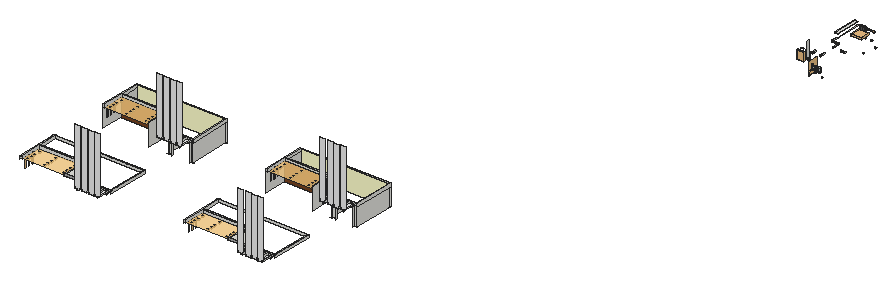
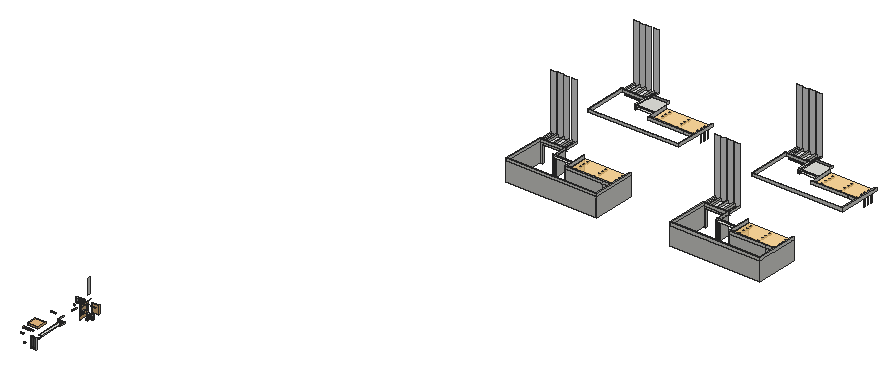
# SketchUp Ruby script. Lengths in inches.
U = 1.inch
M = Sketchup.active_model
def pt(a) = Geom::Point3d.new(a.map { |v| v * U })
def face(e, loops, mat)
  f = e.add_face(loops[0].map { |a| pt(a) })
  loops[1..].each { |l| e.add_face(l.map { |a| pt(a) }).erase! }
  f.material = f.back_material = mat if mat
  f
end
# faces: each face lists its corners as indices into pts; further lists are holes
def faces(e, pts, list, mat = nil) = list.each { |f| face(e, (f[0].is_a?(Array) ? f : [f]).map { |l| l.map { |i| pts[i] } }, mat) }
# xy, xz, yz: faces in a plane at the given z, y or x. An outline is a flat list of corners, or four numbers for a rectangle; further outlines are holes
def ring(l) = l.size == 4 ? [[l[0], l[1]], [l[2], l[1]], [l[2], l[3]], [l[0], l[3]]] : l.each_slice(2).to_a
def flat(e, list, mat, &to3) = list.each { |f| face(e, (f[0].is_a?(Array) ? f : [f]).map { |l| ring(l).map { |u, v| to3.(u, v) } }, mat) }
def xy(e, z, list, mat = nil) = flat(e, list, mat) { |x, y| [x, y, z] }
def xz(e, y, list, mat = nil) = flat(e, list, mat) { |x, z| [x, y, z] }
def yz(e, x, list, mat = nil) = flat(e, list, mat) { |y, z| [x, y, z] }
def lines(e, pts, list) = list.each { |a, b| e.add_line(pt(pts[a]), pt(pts[b])) }
# prism: a flat outline (further loops are holes) pulled along v
def prism(e, loops, v, mat = nil)
  f = face(e, loops, mat); d = Geom::Vector3d.new(v.map { |x| x * U })
  f.pushpull(f.normal.samedirection?(d) ? d.length : -d.length)
end
def box(e, o, s, mat = nil) = prism(e, [[o, [o[0] + s[0], o[1], o[2]], [o[0] + s[0], o[1] + s[1], o[2]], [o[0], o[1] + s[1], o[2]]]], [0, 0, s[2]], mat)
def at(x, y, z, deg = 0) = Geom::Transformation.translation(pt([x, y, z])) * Geom::Transformation.rotation(ORIGIN, Z_AXIS, deg.degrees)
def axes(o, x, y, z) = Geom::Transformation.new([*x, 0, *y, 0, *z, 0, *pt(o).to_a, 1])
def part(name) = M.definitions.add(name)
# library, detail: a bought-in or finely detailed component or shape, given as its bounding box
def library(name, o, s) = part(name).tap { |d| box(d.entities, o, s) }
def detail(e, o, s) = box(e.add_group.entities, o, s)
def put(e, d, t, mat = nil) = e.add_instance(d, t).tap { |i| i.material = mat if mat }
def group(e, t, mat = nil) = e.add_group.tap { |g| g.transformation = t; g.material = mat if mat }.entities
root = M.entities
M.materials.add("6").color = [185, 185, 185]
M.materials.add("WB Frame").color = [245, 245, 245]
M.materials.add("WB Glazing").color = [200, 200, 200]
M.materials["WB Glazing"].alpha = 0.15
M.materials.add("Wood 44").color = [144, 117, 87]
M.materials.add("X22").color = [195, 196, 193]
M.materials.add("[0032_Moccasin]1").color = [255, 228, 181]
M.materials.add("[Carrera Marble]").color = [237, 237, 237]
M.materials.add("[Color E01]").color = [255, 255, 204]
M.materials.add("[Color M03]1").color = [170, 170, 170]
M.materials.add("[Color M08]4").color = [30, 30, 30]
M.materials.add("[Wood Cherry Original]").color = [117, 66, 32]
M.materials.add("[Wood OSB]").color = [255, 207, 129]
M.materials["[Wood OSB]"].alpha = 0.8
M.materials.add("download (88)").color = [169, 176, 150]
c1 = library("Group\#540",[0,0,0],[0.4,67,26])
c2 = part("Window Sliding Main Frame\#3")
prism(c2.entities,[[[35,0,0],[0,0,0],[0,65,0],[35,65,0]],[[1.5,1.5,0],[33.5,1.5,0],[33.5,63.5,0],[1.5,63.5,0]]],[0,0,2.5])
c3 = part("Group428\#1")
xy(c3.entities,0.5,[[3,3,16.75,62]])
c4 = part("Group429\#1")
xy(c4.entities,0.89,[[3,3,16.75,62]])
c5 = part("Window Sliding Casement\#6")
prism(c5.entities,[[[18.25,1.5,0],[1.5,1.5,0],[1.5,63.5,0],[18.25,63.5,0]],[[3,3,0],[16.75,3,0],[16.75,62,0],[3,62,0]]],[0,0,1])
put(c5.entities,c3,at(0,0,0),"WB Glazing")
put(c5.entities,c4,at(0,0,0),"WB Glazing")
c6 = part("Window Sliding Casement\#7")
prism(c6.entities,[[[18.25,1.5,0],[1.5,1.5,0],[1.5,63.5,0],[18.25,63.5,0]],[[3,3,0],[16.75,3,0],[16.75,62,0],[3,62,0]]],[0,0,1])
put(c6.entities,c3,at(0,0,0),"WB Glazing")
put(c6.entities,c4,at(0,0,0),"WB Glazing")
c7 = part("Window Sliding\#3")
put(c7.entities,c2,at(0,0,0),"WB Frame")
put(c7.entities,c5,at(0,0,0),"WB Frame")
put(c7.entities,c6,at(15.25,0,1),"WB Frame")
c8 = library("Group\#467",[0,0,0],[8.82,3.39,0.43])
c9 = library("Group\#465",[0,0,0],[8.82,3.39,0.43])
c10 = library("Group\#488",[0,0,0],[8.82,3.39,0.43])
c11 = library("Group\#466",[0,0,0],[8.82,3.39,0.43])
c12 = library("Group\#541",[0,0,0],[0.4,67,50])
c13 = library("Group\#468",[0,0,0],[8.82,3.39,0.43])
c14 = part("Group\#543")
prism(c14.entities,[[[4.74,0,0],[4.74,0,2.625],[0,0,2.625],[0,0,1.6875],[4.25,0,1.6875],[4.25,0,0]]],[0,1.25,0])
c15 = library("Vase of roses",[-3.61,-2.29,-1.14],[22.21,22.69,31.56])
c16 = part("X1")
xy(c16.entities,0.79,[[292.49,554.16,383.77,683.125],[106.61,647.12,250.85,858.41],[424.25,648.04,568.45,857.91],[293.37,729.03,384.53,857.56]],"X22")
xy(c16.entities,0.79,[[[281.2,542.875,395.06,694.41],[292.49,554.16,383.77,683.125]],[[95.33,635.84,262.14,869.69],[106.61,647.12,250.85,858.41]],[[412.97,636.75,579.74,869.19],[424.25,648.04,568.45,857.91]],[[282.08,717.74,395.82,868.85],[293.37,729.03,384.53,857.56]]],"[Color M08]4")
xz(c16.entities,542.875,[[281.2,-12.48,395.06,0.79]],"X22")
xz(c16.entities,635.84,[[95.33,-12.48,262.14,0.79]],"X22")
xz(c16.entities,636.75,[[412.97,-12.48,579.74,0.79]],"X22")
xz(c16.entities,694.41,[[281.2,-12.48,395.06,0.79]],"X22")
xz(c16.entities,717.74,[[282.08,-12.48,395.82,0.79]],"X22")
xz(c16.entities,868.85,[[282.08,-12.48,395.82,0.79]],"X22")
xz(c16.entities,869.19,[[412.97,-12.48,579.74,0.79]],"X22")
xz(c16.entities,869.69,[[95.33,-12.48,262.14,0.79]],"X22")
yz(c16.entities,95.33,[[635.84,-12.48,869.69,0.79]],"X22")
yz(c16.entities,262.14,[[635.84,-12.48,869.69,0.79]],"[Color M08]4")
yz(c16.entities,281.2,[[542.875,-12.48,694.41,0.79]],"X22")
yz(c16.entities,282.08,[[717.74,-12.48,868.85,0.79]],"X22")
yz(c16.entities,395.06,[[542.875,-12.48,694.41,0.79]],"X22")
yz(c16.entities,395.82,[[717.74,-12.48,868.85,0.79]],"X22")
yz(c16.entities,412.97,[[636.75,-12.48,869.19,0.79]],"X22")
yz(c16.entities,579.74,[[636.75,-12.48,869.19,0.79]],"X22")
c17 = part("Framed Art Print 001")
xy(c17.entities,0,[[-4.59,-0.26,-4.59,0.26,4.59,0.26],[-4.59,-0.26,4.59,0.26,4.59,-0.26]])
xy(c17.entities,12.66,[[-4.59,-0.26,4.59,-0.26,-4.59,0.26],[4.59,-0.26,4.59,0.26,-4.59,0.26]])
xz(c17.entities,-0.26,[[-4.59,0,4.59,0,-4.59,12.66],[4.59,0,4.59,12.66,-4.59,12.66]])
xz(c17.entities,0.26,[[-4.59,0,-4.59,12.66,4.59,12.66],[-4.59,0,4.59,12.66,4.59,0]])
yz(c17.entities,-4.59,[[-0.26,0,-0.26,12.66,0.26,0],[0.26,0,-0.26,12.66,0.26,12.66]])
yz(c17.entities,4.59,[[-0.26,0,0.26,0,-0.26,12.66],[0.26,0,0.26,12.66,-0.26,12.66]])
c18 = library("Group\#528",[0,-11.75,0],[9,47,61.5])
c19 = library("Component\#3",[0,0,0],[1.18,41.92,1.7])
c20 = part("Group\#487")
box(c20.entities,[0,0,0],[4,4,4])
c21 = library("Group\#506",[75.42,83.05,1.23],[65.76,64.05,12.4])
c22 = library("Light+Luminária+Spot+Control",[-53.76,-1.97,-0.51],[47.25,4.73,6.22])
c23 = part("Group\#530")
box(c23.entities,[0,0,0],[0.5,24,0.1])
c24 = library("A$C06767DEF\#1",[-8.3,1.21,0],[7.09,7.09,5.51])
xy(root,115.81,[[647.46,387.84,757.46,394.91],[1695.77,387.84,1805.77,394.91]])
xy(root,120.25,[[647.11,1046.93,757.11,1054],[1695.43,1046.93,1805.43,1054]])
xy(root,126.75,[[208.91,387.84,486.41,528.53],[1257.22,387.84,1534.73,528.53]],"[Wood OSB]")
xy(root,131.1875,[[208.57,1046.93,486.07,1187.62],[1256.88,1046.93,1534.38,1187.62]],"[Wood OSB]")
xy(root,133.625,[[626.68,309.65,641.55,387.84],[657.03,309.65,689.24,387.84],[698.65,309.65,730.86,387.84],[739.28,309.65,761.74,387.84],[1674.99,309.65,1689.86,387.84],
  [1705.34,309.65,1737.55,387.84],[1746.96,309.65,1779.17,387.84],[1787.59,309.65,1810.05,387.84]],"[Carrera Marble]")
xy(root,136.875,[[609.34,309.65,626.68,387.84],[1657.65,309.65,1674.99,387.84]])
xy(root,138,[[500.81,477.09,607.63,494.59],[1549.12,477.09,1655.94,494.59]])
xy(root,138.0625,[[626.34,968.74,641.2,1046.93],[656.68,968.74,688.89,1046.93],[698.31,968.74,730.52,1046.93],[738.93,968.74,761.39,1046.93],[1674.65,968.74,1689.52,1046.93],
  [1705,968.74,1737.2,1046.93],[1746.62,968.74,1778.83,1046.93],[1787.25,968.74,1809.71,1046.93]],"[Carrera Marble]")
xy(root,138.5625,[[609.09,398.1,615.97,448.72],[615.97,398.1,626.68,448.72],[1657.41,398.1,1664.28,448.72],[1664.28,398.1,1674.99,448.72]])
xy(root,139.5,[[761.74,309.65,771.49,387.84],[1810.05,309.65,1819.8,387.84]])
xy(root,141.3125,[[609,968.74,626.34,1046.93],[1657.31,968.74,1674.65,1046.93]])
xy(root,142.4375,[[500.46,1136.18,607.28,1153.68],[1548.77,1136.18,1655.6,1153.68]])
xy(root,143,[[608.75,1057.1875,615.625,1107.8125],[615.625,1057.1875,626.34,1107.8125],[1657.0625,1057.1875,1663.9375,1107.8125],[1663.9375,1057.1875,1674.65,1107.8125]])
xy(root,143.9375,[[761.39,968.74,771.14,1046.93],[1809.71,968.74,1819.45,1046.93]])
xy(root,144.3125,[[497.6,365.47,497.6,387.84,499.53,387.84,499.53,477.09,609.09,477.09,609.09,365.47],[609.09,365.47,626.68,387.84],[1545.92,365.47,1545.92,387.84,1547.84,387.84,1547.84,477.09,1657.41,477.09,1657.41,365.47],[1657.41,365.47,1674.99,387.84],[609.09,387.84,626.68,387.84,626.68,394.91,616.45,394.91,616.45,477.09,609.09,477.09],
  [1657.41,387.84,1674.99,387.84,1674.99,394.91,1664.77,394.91,1664.77,477.09,1657.41,477.09],[616.45,394.91,626.68,477.09],[1664.77,394.91,1674.99,477.09],[607.63,477.09,616.45,494.59],[1655.94,477.09,1664.77,494.59]])
xz(root,309.65,[[626.68,133.625,641.55,133.625,641.55,502.82,609.34,502.82,609.34,136.875,626.68,136.875],[657.03,133.625,689.24,502.82],[698.65,133.625,730.86,502.82],[739.28,133.625,761.74,133.625,761.74,139.5,771.49,139.5,771.49,502.82,739.28,502.82],[1674.99,133.625,1689.86,133.625,1689.86,502.82,1657.65,502.82,1657.65,136.875,1674.99,136.875],
  [1705.34,133.625,1737.55,502.82],[1746.96,133.625,1779.17,502.82],[1787.59,133.625,1810.05,133.625,1810.05,139.5,1819.8,139.5,1819.8,502.82,1787.59,502.82]],"[Carrera Marble]")
xz(root,365.47,[[609.09,144.3125,626.68,144.9375],[1657.41,144.3125,1674.99,144.9375]])
xz(root,365.47,[[497.6,144.3125,609.09,157.5],[1545.92,144.3125,1657.41,157.5]],"[Color M03]1")
xz(root,387.84,[[626.68,133.625,641.55,144.3125],[657.03,133.625,689.24,144.3125],[698.65,133.625,730.86,144.3125],[739.28,133.625,761.74,133.625,761.74,139.5,771.49,139.5,771.49,144.3125,739.28,144.3125],[1674.99,133.625,1689.86,144.3125],
  [1705.34,133.625,1737.55,144.3125],[1746.96,133.625,1779.17,144.3125],[1787.59,133.625,1810.05,133.625,1810.05,139.5,1819.8,139.5,1819.8,144.3125,1787.59,144.3125],[609.34,136.875,626.68,144.3125],[1657.65,136.875,1674.99,144.3125],
  [609.09,144.3125,609.34,144.9375],[609.34,144.3125,626.68,144.9375],[626.68,144.3125,641.55,144.9375],[641.55,144.3125,657.03,144.9375],[689.24,144.3125,698.65,144.9375],
  [730.86,144.3125,739.28,144.9375],[771.49,144.3125,782.78,144.9375],[1657.41,144.3125,1657.65,144.9375],[1657.65,144.3125,1674.99,144.9375],[1674.99,144.3125,1689.86,144.9375],
  [1689.86,144.3125,1705.34,144.9375],[1737.55,144.3125,1746.96,144.9375],[1779.17,144.3125,1787.59,144.9375],[1819.8,144.3125,1831.09,144.9375]])
xz(root,394.91,[[493.2,126.75,497.6,144.3125],[616.45,126.75,775.16,144.3125],[1541.52,126.75,1545.92,144.3125],[1664.77,126.75,1823.47,144.3125]])
xz(root,477.09,[[499.53,126.75,500.81,144.3125],[607.63,126.75,609.09,144.3125],[609.09,126.75,626.68,144.3125],[1547.84,126.75,1549.12,144.3125],[1655.94,126.75,1657.41,144.3125],
  [1657.41,126.75,1674.99,144.3125],[500.81,138,607.63,144.3125],[1549.12,138,1655.94,144.3125]])
xz(root,494.59,[[499.53,126.75,500.81,144.3125],[607.63,126.75,616.45,144.3125],[1547.84,126.75,1549.12,144.3125],[1655.94,126.75,1664.77,144.3125]])
xz(root,528.53,[[208.91,126.75,493.2,144.3125],[1257.22,126.75,1541.52,144.3125]])
xz(root,538.16,[[208.91,126.75,262.79,144.3125],[262.79,126.75,499.53,144.3125],[1257.22,126.75,1311.1,144.3125],[1311.1,126.75,1547.84,144.3125]])
xz(root,659.09,[[200.03,126.75,782.78,144.3125],[1248.34,126.75,1831.09,144.3125],[200.03,144.3125,782.78,144.9375],[1248.34,144.3125,1831.09,144.9375]])
xz(root,968.74,[[626.34,138.0625,641.2,138.0625,641.2,507.25,609,507.25,609,141.3125,626.34,141.3125],[656.68,138.0625,688.89,507.25],[698.31,138.0625,730.52,507.25],[738.93,138.0625,761.39,138.0625,761.39,143.9375,771.14,143.9375,771.14,507.25,738.93,507.25],[1674.65,138.0625,1689.52,138.0625,1689.52,507.25,1657.31,507.25,1657.31,141.3125,1674.65,141.3125],
  [1705,138.0625,1737.2,507.25],[1746.62,138.0625,1778.83,507.25],[1787.25,138.0625,1809.71,138.0625,1809.71,143.9375,1819.45,143.9375,1819.45,507.25,1787.25,507.25]],"[Carrera Marble]")
xz(root,1046.93,[[626.34,138.0625,641.2,148.75],[656.68,138.0625,688.89,148.75],[698.31,138.0625,730.52,148.75],[738.93,138.0625,761.39,138.0625,761.39,143.9375,771.14,143.9375,771.14,148.75,738.93,148.75],[1674.65,138.0625,1689.52,148.75],
  [1705,138.0625,1737.2,148.75],[1746.62,138.0625,1778.83,148.75],[1787.25,138.0625,1809.71,138.0625,1809.71,143.9375,1819.45,143.9375,1819.45,148.75,1787.25,148.75],[609,141.3125,626.34,148.75],[1657.31,141.3125,1674.65,148.75]])
xz(root,1054,[[616.11,11.1875,616.11,131.1875,774.8125,131.1875,774.8125,11.1875,757.11,11.1875,757.11,120.25,647.11,120.25,647.11,11.1875],[1664.42,11.1875,1664.42,131.1875,1823.125,131.1875,1823.125,11.1875,1805.43,11.1875,1805.43,120.25,1695.43,120.25,1695.43,11.1875],[492.86,131.1875,497.26,148.75],[616.11,131.1875,774.8125,148.75],[1541.17,131.1875,1545.57,148.75],
  [1664.42,131.1875,1823.125,148.75]])
xz(root,1136.18,[[499.1875,11.1875,500.46,131.1875],[607.28,11.1875,608.75,131.1875],[608.75,11.1875,626.34,131.1875],[1547.5,11.1875,1548.77,131.1875],[1655.6,11.1875,1657.0625,131.1875],
  [1657.0625,11.1875,1674.65,131.1875],[499.1875,131.1875,500.46,148.75],[607.28,131.1875,608.75,148.75],[608.75,131.1875,626.34,148.75],[1547.5,131.1875,1548.77,148.75],
  [1655.6,131.1875,1657.0625,148.75],[1657.0625,131.1875,1674.65,148.75],[500.46,142.4375,607.28,148.75],[1548.77,142.4375,1655.6,148.75]])
xz(root,1153.68,[[499.1875,11.1875,500.46,131.1875],[607.28,11.1875,616.11,131.1875],[1547.5,11.1875,1548.77,131.1875],[1655.6,11.1875,1664.42,131.1875],[499.1875,131.1875,500.46,148.75],
  [607.28,131.1875,616.11,148.75],[1547.5,131.1875,1548.77,148.75],[1655.6,131.1875,1664.42,148.75]])
xz(root,1187.62,[[486.07,11.1875,492.86,131.1875],[1534.38,11.1875,1541.17,131.1875],[208.57,131.1875,492.86,148.75],[1256.88,131.1875,1541.17,148.75]])
xz(root,1187.62,[[208.57,11.1875,486.07,131.1875],[1256.88,11.1875,1534.38,131.1875]],"[Wood Cherry Original]")
xz(root,1197.25,[[208.57,11.1875,262.44,131.1875],[262.44,11.1875,499.1875,131.1875],[1256.88,11.1875,1310.75,131.1875],[1310.75,11.1875,1547.5,131.1875],[208.57,131.1875,262.44,148.75],
  [262.44,131.1875,499.1875,148.75],[1256.88,131.1875,1310.75,148.75],[1310.75,131.1875,1547.5,148.75]])
xz(root,1311.11,[[208.57,11.1875,774.8125,148.75],[1256.88,11.1875,1823.125,148.75]],"[Color E01]")
xz(root,1318.18,[[199.6875,11.1875,782.4375,131.1875],[1248,11.1875,1830.75,131.1875],[199.6875,131.1875,782.4375,148.75],[1248,131.1875,1830.75,148.75]])
yz(root,199.6875,[[1046.93,11.1875,1318.18,131.1875],[1046.93,131.1875,1318.18,148.75]])
yz(root,200.03,[[387.84,126.75,659.09,144.3125],[387.84,144.3125,659.09,144.9375]])
yz(root,208.57,[[1197.25,11.1875,1311.11,131.1875],[1054,131.1875,1187.62,148.75],[1197.25,131.1875,1311.11,148.75]])
yz(root,208.91,[[394.91,126.75,528.53,144.3125],[538.16,126.75,652.02,144.3125]])
yz(root,492.86,[[1054,131.1875,1187.62,148.75]])
yz(root,493.2,[[394.91,126.75,528.53,144.3125]])
yz(root,497.6,[[365.47,144.3125,387.84,157.5]])
yz(root,499.1875,[[1046.93,11.1875,1136.18,148.75],[1153.68,11.1875,1197.25,148.75]])
yz(root,500.46,[[1136.18,11.1875,1153.68,142.4375],[1136.18,142.4375,1153.68,148.75]])
yz(root,500.81,[[477.09,138,494.59,144.3125]])
yz(root,607.28,[[1136.18,142.4375,1153.68,148.75]])
yz(root,607.63,[[477.09,138,494.59,144.3125]])
yz(root,609,[[968.74,141.3125,1046.93,149.375]])
yz(root,609.09,[[365.47,144.3125,387.84,144.9375],[387.84,144.3125,389.4,144.9375]])
yz(root,609.34,[[309.65,136.875,387.84,144.9375]])
yz(root,616.11,[[1054,11.1875,1153.68,131.1875],[1054,131.1875,1153.68,148.75]])
yz(root,616.45,[[394.91,126.75,494.59,144.3125]])
yz(root,626.34,[[968.74,138.0625,1000.12,141.3125],[1000.12,138.0625,1046.93,141.3125],[1046.93,138.0625,1048.49,141.3125],[1000.12,141.3125,1046.93,141.3125,1046.93,148.75,1024.56,148.75,1024.56,149.375,1000.12,149.375],[1046.93,141.3125,1048.49,148.75]])
yz(root,626.68,[[309.65,133.625,341.03,136.875],[341.03,133.625,387.84,136.875],[387.84,133.625,389.4,136.875],[341.03,136.875,387.84,136.875,387.84,144.3125,365.47,144.3125,365.47,144.9375,341.03,144.9375],[387.84,136.875,389.4,144.3125],
  [365.47,144.3125,387.84,144.9375],[387.84,144.3125,389.4,144.9375]])
yz(root,641.2,[[968.74,138.0625,1046.93,149.375]])
yz(root,641.55,[[309.65,133.625,387.84,144.9375]])
yz(root,647.11,[[1046.93,11.1875,1054,120.25]])
yz(root,656.68,[[968.74,138.0625,1046.93,149.375]])
yz(root,657.03,[[309.65,133.625,387.84,144.9375]])
yz(root,688.89,[[968.74,138.0625,1046.93,149.375]])
yz(root,689.24,[[309.65,133.625,387.84,144.9375]])
yz(root,698.31,[[968.74,138.0625,1046.93,149.375]])
yz(root,698.65,[[309.65,133.625,387.84,144.9375]])
yz(root,730.52,[[968.74,138.0625,1046.93,149.375]])
yz(root,730.86,[[309.65,133.625,387.84,144.9375]])
yz(root,738.93,[[968.74,138.0625,1046.93,149.375]])
yz(root,739.28,[[309.65,133.625,387.84,144.9375]])
yz(root,757.11,[[1046.93,11.1875,1054,120.25]])
yz(root,761.39,[[968.74,138.0625,1046.93,143.9375]])
yz(root,761.74,[[309.65,133.625,387.84,139.5]])
yz(root,771.14,[[968.74,143.9375,1046.93,149.375]])
yz(root,771.49,[[309.65,139.5,387.84,144.9375]])
yz(root,774.8125,[[1054,11.1875,1311.11,131.1875],[1054,131.1875,1311.11,148.75]])
yz(root,775.16,[[394.91,126.75,652.02,144.3125]])
yz(root,782.4375,[[1046.93,131.1875,1318.18,148.75]])
yz(root,782.78,[[387.84,126.75,659.09,144.3125],[387.84,144.3125,659.09,144.9375]])
yz(root,1248,[[1046.93,11.1875,1318.18,131.1875],[1046.93,131.1875,1318.18,148.75]])
yz(root,1248.34,[[387.84,126.75,659.09,144.3125],[387.84,144.3125,659.09,144.9375]])
yz(root,1256.88,[[1197.25,11.1875,1311.11,131.1875],[1054,131.1875,1187.62,148.75],[1197.25,131.1875,1311.11,148.75]])
yz(root,1257.22,[[394.91,126.75,528.53,144.3125],[538.16,126.75,652.02,144.3125]])
yz(root,1541.17,[[1054,131.1875,1187.62,148.75]])
yz(root,1541.52,[[394.91,126.75,528.53,144.3125]])
yz(root,1545.92,[[365.47,144.3125,387.84,157.5]])
yz(root,1547.5,[[1046.93,11.1875,1136.18,148.75],[1153.68,11.1875,1197.25,148.75]])
yz(root,1548.77,[[1136.18,11.1875,1153.68,142.4375],[1136.18,142.4375,1153.68,148.75]])
yz(root,1549.12,[[477.09,138,494.59,144.3125]])
yz(root,1655.6,[[1136.18,142.4375,1153.68,148.75]])
yz(root,1655.94,[[477.09,138,494.59,144.3125]])
yz(root,1657.31,[[968.74,141.3125,1046.93,149.375]])
yz(root,1657.41,[[365.47,144.3125,387.84,144.9375],[387.84,144.3125,389.4,144.9375]])
yz(root,1657.65,[[309.65,136.875,387.84,144.9375]])
yz(root,1664.42,[[1054,11.1875,1153.68,131.1875],[1054,131.1875,1153.68,148.75]])
yz(root,1664.77,[[394.91,126.75,494.59,144.3125]])
yz(root,1674.65,[[968.74,138.0625,1000.12,141.3125],[1000.12,138.0625,1046.93,141.3125],[1046.93,138.0625,1048.49,141.3125],[1000.12,141.3125,1046.93,141.3125,1046.93,148.75,1024.56,148.75,1024.56,149.375,1000.12,149.375],[1046.93,141.3125,1048.49,148.75]])
yz(root,1674.99,[[309.65,133.625,341.03,136.875],[341.03,133.625,387.84,136.875],[387.84,133.625,389.4,136.875],[341.03,136.875,387.84,136.875,387.84,144.3125,365.47,144.3125,365.47,144.9375,341.03,144.9375],[387.84,136.875,389.4,144.3125],
  [365.47,144.3125,387.84,144.9375],[387.84,144.3125,389.4,144.9375]])
yz(root,1689.52,[[968.74,138.0625,1046.93,149.375]])
yz(root,1689.86,[[309.65,133.625,387.84,144.9375]])
yz(root,1695.43,[[1046.93,11.1875,1054,120.25]])
yz(root,1705,[[968.74,138.0625,1046.93,149.375]])
yz(root,1705.34,[[309.65,133.625,387.84,144.9375]])
yz(root,1737.2,[[968.74,138.0625,1046.93,149.375]])
yz(root,1737.55,[[309.65,133.625,387.84,144.9375]])
yz(root,1746.62,[[968.74,138.0625,1046.93,149.375]])
yz(root,1746.96,[[309.65,133.625,387.84,144.9375]])
yz(root,1778.83,[[968.74,138.0625,1046.93,149.375]])
yz(root,1779.17,[[309.65,133.625,387.84,144.9375]])
yz(root,1787.25,[[968.74,138.0625,1046.93,149.375]])
yz(root,1787.59,[[309.65,133.625,387.84,144.9375]])
yz(root,1805.43,[[1046.93,11.1875,1054,120.25]])
yz(root,1809.71,[[968.74,138.0625,1046.93,143.9375]])
yz(root,1810.05,[[309.65,133.625,387.84,139.5]])
yz(root,1819.45,[[968.74,143.9375,1046.93,149.375]])
yz(root,1819.8,[[309.65,139.5,387.84,144.9375]])
yz(root,1823.125,[[1054,11.1875,1311.11,131.1875],[1054,131.1875,1311.11,148.75]])
yz(root,1823.47,[[394.91,126.75,652.02,144.3125]])
yz(root,1830.75,[[1046.93,131.1875,1318.18,148.75]])
yz(root,1831.09,[[387.84,126.75,659.09,144.3125],[387.84,144.3125,659.09,144.9375]])
p = [[609.09,387.84,126.75],[626.68,387.84,126.75],[208.91,394.91,144.3125],[208.91,387.84,144.3125],[493.2,394.91,126.75],[493.2,387.84,126.75],
  [497.6,394.91,144.3125],[497.6,387.84,144.3125],[1257.22,394.91,144.3125],[1257.22,387.84,144.3125],[1657.41,387.84,126.75],[1674.99,387.84,126.75],
  [1541.52,394.91,126.75],[1541.52,387.84,126.75],[1545.92,394.91,144.3125],[1545.92,387.84,144.3125],[782.4375,1054,11.1875],[774.8125,1054,11.1875],
  [262.44,1197.25,11.1875],[262.44,1187.62,11.1875],[782.4375,1311.11,11.1875],[774.8125,1311.11,11.1875],[782.4375,1318.18,11.1875],[608.75,1046.93,11.1875],
  [626.34,1046.93,11.1875],[608.75,1046.93,131.1875],[626.34,1046.93,131.1875],[492.86,1054,131.1875],[492.86,1046.93,131.1875],[1830.75,1054,11.1875],
  [1823.125,1054,11.1875],[1310.75,1197.25,11.1875],[1310.75,1187.62,11.1875],[1830.75,1311.11,11.1875],[1830.75,1318.18,11.1875],[1657.0625,1046.93,11.1875],
  [1674.65,1046.93,11.1875],[1823.125,1311.11,11.1875],[1657.0625,1046.93,131.1875],[1674.65,1046.93,131.1875],[1541.17,1054,131.1875],[1541.17,1046.93,131.1875]]
lines(root,p,[[0,1],[2,3],[4,5],[6,7],[8,9],[10,11],[12,13],[14,15],[16,17],[18,19],[20,21],[20,22],
  [23,24],[25,26],[27,28],[29,30],[31,32],[33,34],[35,36],[33,37],[38,39],[40,41]])
put(root,c1,at(2620.7,3681.75,8))
put(root,c1,axes([2620.76,3685.75,12],[0.85,0,0],[0,0.8806,0],[0,0,0.69231]))
put(root,c7,axes([2622.1,4135.25,22],[-1,0,0],[0,0,1],[0,1,0]))
put(root,c8,axes([2709.35,4002.67,26.4],[1,0,0],[0,0,1],[0,1,0]),"Wood 44")
put(root,c9,axes([2662.49,4128.75,27.19],[1,0,0],[0,0,1],[0,-1,0]),"Wood 44")
put(root,c10,axes([2564.28,3755.94,30],[1,0,0],[0,0,1],[0,-1,0]))
put(root,c11,axes([2708.28,3675.94,30],[1,0,0],[0,0,1],[0,-1,0]),"Wood 44")
put(root,c12,at(2620.7,3681.75,35))
put(root,c13,axes([2731.52,4069.75,35.14],[1,0,0],[0,0,1],[0,1,0]),"Wood 44")
put(root,c8,axes([2732.92,4070.75,35.72],[1,0,0],[0,0,1],[0,1,0]),"Wood 44")
put(root,c14,at(2616.36,3725.98,36.31))
put(root,c14,at(2616.36,3703.1,36.31))
put(root,c15,axes([2613.87,3711.5,38.51],[0.3886,0,0],[0,0.3886,0],[0,0,0.3886]))
g1 = group(root,at(2615.1,3700.75,38.17))
prism(g1,[[[5.95,29,0],[5.95,0,0],[1.7,0,0],[1.48,0.02,0],[1.26,0.07,0],[1.05,0.15,0],[0.85,0.27,0],[0.67,0.41,0],[0.5,0.59,0],[0.35,0.78,0],[0.23,1,0],[0.13,1.23,0],[0.06,1.48,0],[0.01,1.74,0],[0,2,0],[0,27,0],[0.01,27.26,0],[0.06,27.52,0],[0.13,27.77,0],[0.23,28,0],[0.35,28.22,0],[0.5,28.41,0],[0.67,28.59,0],[0.85,28.73,0],[1.05,28.85,0],[1.26,28.93,0],[1.48,28.98,0],[1.7,29,0]]],[0,0,0.52])
g2 = group(root,at(2620.6,3688.75,41.7))
yz(g2,0,[[0.5,0.5,52.5,35.5]],"WB Glazing")
g3 = group(g2,at(0,0,0))
xy(g3,0,[[0,0,0.5,53]],"6")
xy(g3,0.5,[[0,0.5,0.25,52.5]],"6")
xy(g3,35.5,[[0,0.5,0.25,52.5]],"6")
xy(g3,36,[[0,0,0.5,53]],"6")
xz(g3,0,[[0,0,0.5,36]],"6")
xz(g3,0.5,[[0,0.5,0.25,35.5]],"6")
xz(g3,52.5,[[0,0.5,0.25,35.5]],"6")
xz(g3,53,[[0,0,0.5,36]],"6")
yz(g3,0,[[[0,0,53,36],[0.5,0.5,52.5,35.5]]],"6")
yz(g3,0.5,[[0,0,53,36]],"6")
g4 = group(g2,at(0.25,0.5,0.5),"WB Glazing")
yz(g4,0,[[0,0,52,35]],"download (88)")
put(root,c16,axes([2631.17,3676.52,-21.4],[0.12,0,0],[0,0,0.12],[0,-0.018,0]))
put(root,c17,axes([2558.54,3755.55,45.375],[2.19,0,0],[0,0.7884,0],[0,0,2.19]))
put(root,c17,axes([2533.67,3755.55,45.375],[2.19,0,0],[0,0.7884,0],[0,0,2.19]))
put(root,c18,axes([2534.41,3716.78,108.92],[0,-1.33292,0],[1,0,0],[0,0,-0.782]))
put(root,c19,axes([208.91,414.82,130.83],[0,-1,0],[0,0,-1.54],[1,0,0]))
put(root,c19,axes([208.91,442.82,130.83],[0,-1,0],[0,0,-1.54],[1,0,0]))
put(root,c19,axes([208.91,472.57,130.83],[0,-1,0],[0,0,-1.54],[1,0,0]))
put(root,c19,axes([1257.22,414.82,130.83],[0,-1,0],[0,0,-1.54],[1,0,0]))
put(root,c19,axes([1257.22,442.82,130.83],[0,-1,0],[0,0,-1.54],[1,0,0]))
put(root,c19,axes([1257.22,472.57,130.83],[0,-1,0],[0,0,-1.54],[1,0,0]))
put(root,c19,axes([208.57,1073.91,135.27],[0,-1,0],[0,0,-1.54],[1,0,0]))
put(root,c19,axes([208.57,1101.91,135.27],[0,-1,0],[0,0,-1.54],[1,0,0]))
put(root,c19,axes([208.57,1131.66,135.27],[0,-1,0],[0,0,-1.54],[1,0,0]))
put(root,c19,axes([1256.88,1073.91,135.27],[0,-1,0],[0,0,-1.54],[1,0,0]))
put(root,c19,axes([1256.88,1101.91,135.27],[0,-1,0],[0,0,-1.54],[1,0,0]))
put(root,c19,axes([1256.88,1131.66,135.27],[0,-1,0],[0,0,-1.54],[1,0,0]))
put(root,c9,axes([2672.34,4131.75,79.41],[1,0,0],[0,0,1],[0,-1,0]),"Wood 44")
put(root,c20,axes([2581.1,3918.75,83],[9.25,0,0],[0,1.5,0],[0,0,1]))
put(root,c20,axes([2674.06,3868.75,83],[6.76,0,0],[0,1.5,0],[0,0,1]))
put(root,c20,axes([2621.1,3765.75,83],[1.5,0,0],[0,9,0],[0,0,1]))
put(root,c20,axes([2621.1,3874.75,83],[1.25,0,0],[0,9.25,0],[0,0,1]))
put(root,c20,axes([2573.1,3764.75,83],[1.5,0,0],[0,7,0],[0,0,1]))
put(root,c20,axes([2573.1,3928.75,83],[1.5,0,0],[0,7,0],[0,0,1]))
g5 = group(root,at(2578.1,3967.75,84.2))
box(g5,[0,0,0],[0.75,161,1.1])
put(root,c21,at(2555.1,3924.75,94),"Wood 44")
put(root,c22,at(2700.23,4106.59,98.1875))
g6 = group(root,at(2555.1,3967.75,0))
g7 = group(g6,at(0.125,0,104.0625))
xy(g7,0,[[0,0,23.625,161]])
xy(g7,3.9375,[[0,0,23.625,161]])
xz(g7,0,[[0,0,23.625,3.9375]])
xz(g7,161,[[0,0,23.625,3.9375]])
yz(g7,0,[[0,0,161,3.9375]])
yz(g7,23.625,[[0,0,161,3.9375]],"Wood 44")
put(root,c23,axes([2598.6,3686.75,109.9],[1,0,0],[0,2.375,0],[0,0,1]),"[0032_Moccasin]1")
put(root,c23,axes([2523.1,3737.78,109.9],[0,-1,0],[3.66667,0,0],[0,0,1]),"[0032_Moccasin]1")
g8 = group(root,at(2624.1,3657.75,120.91))
yz(g8,0,[[0,0,18,92.85]])
put(root,c24,at(235.46,497.86,121.24))
put(root,c24,at(235.46,461.74,121.24))
put(root,c24,at(235.46,435.43,121.24))
put(root,c24,at(235.46,407.55,121.24))
put(root,c24,at(342.15,407.55,121.24))
put(root,c24,at(342.15,497.86,121.24))
put(root,c24,at(342.15,435.43,121.24))
put(root,c24,at(342.15,461.74,121.24))
put(root,c24,at(462.77,407.55,121.24))
put(root,c24,at(462.77,497.86,121.24))
put(root,c24,at(462.77,435.43,121.24))
put(root,c24,at(462.77,461.74,121.24))
put(root,c24,at(1390.46,407.55,121.24))
put(root,c24,at(1283.77,407.55,121.24))
put(root,c24,at(1283.77,497.86,121.24))
put(root,c24,at(1283.77,435.43,121.24))
put(root,c24,at(1390.46,497.86,121.24))
put(root,c24,at(1390.46,435.43,121.24))
put(root,c24,at(1390.46,461.74,121.24))
put(root,c24,at(1283.77,461.74,121.24))
put(root,c24,at(1511.09,461.74,121.24))
put(root,c24,at(1511.09,435.43,121.24))
put(root,c24,at(1511.09,407.55,121.24))
put(root,c24,at(1511.09,497.86,121.24))
put(root,c24,at(341.8,1066.64,125.68))
put(root,c24,at(235.12,1066.64,125.68))
put(root,c24,at(235.12,1156.95,125.68))
put(root,c24,at(235.12,1094.52,125.68))
put(root,c24,at(341.8,1156.95,125.68))
put(root,c24,at(341.8,1094.52,125.68))
put(root,c24,at(341.8,1120.83,125.68))
put(root,c24,at(235.12,1120.83,125.68))
put(root,c24,at(462.43,1120.83,125.68))
put(root,c24,at(462.43,1094.52,125.68))
put(root,c24,at(462.43,1066.64,125.68))
put(root,c24,at(462.43,1156.95,125.68))
put(root,c24,at(1510.74,1094.52,125.68))
put(root,c24,at(1510.74,1156.95,125.68))
put(root,c24,at(1510.74,1066.64,125.68))
put(root,c24,at(1283.43,1066.64,125.68))
put(root,c24,at(1283.43,1156.95,125.68))
put(root,c24,at(1283.43,1094.52,125.68))
put(root,c24,at(1390.12,1156.95,125.68))
put(root,c24,at(1390.12,1094.52,125.68))
put(root,c24,at(1390.12,1066.64,125.68))
put(root,c24,at(1390.12,1120.83,125.68))
put(root,c24,at(1283.43,1120.83,125.68))
put(root,c24,at(1510.74,1120.83,125.68))
